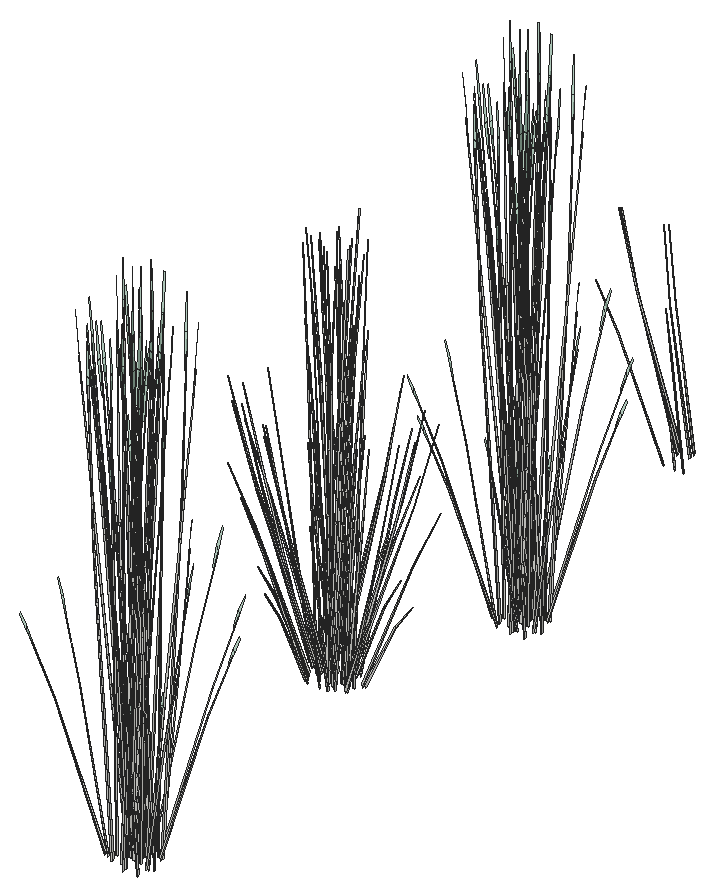
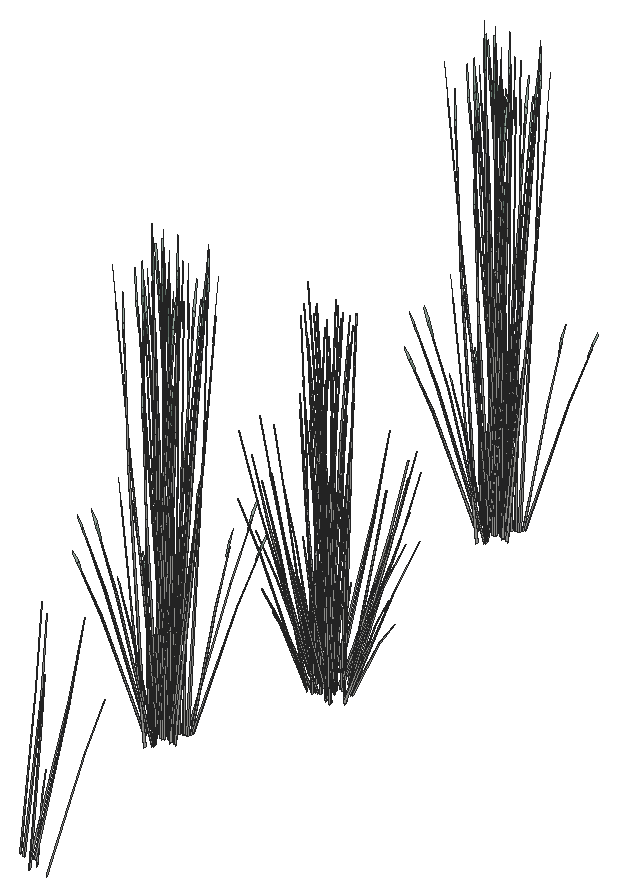
# SketchUp Ruby script. Lengths in inches.
U = 1.inch
M = Sketchup.active_model
def pt(a) = Geom::Point3d.new(a.map { |v| v * U })
def face(e, loops, mat)
  f = e.add_face(loops[0].map { |a| pt(a) })
  loops[1..].each { |l| e.add_face(l.map { |a| pt(a) }).erase! }
  f.material = f.back_material = mat if mat
  f
end
# faces: each face lists its corners as indices into pts; further lists are holes
def faces(e, pts, list, mat = nil) = list.each { |f| face(e, (f[0].is_a?(Array) ? f : [f]).map { |l| l.map { |i| pts[i] } }, mat) }
# xy, xz, yz: faces in a plane at the given z, y or x. An outline is a flat list of corners, or four numbers for a rectangle; further outlines are holes
def ring(l) = l.size == 4 ? [[l[0], l[1]], [l[2], l[1]], [l[2], l[3]], [l[0], l[3]]] : l.each_slice(2).to_a
def flat(e, list, mat, &to3) = list.each { |f| face(e, (f[0].is_a?(Array) ? f : [f]).map { |l| ring(l).map { |u, v| to3.(u, v) } }, mat) }
def xy(e, z, list, mat = nil) = flat(e, list, mat) { |x, y| [x, y, z] }
def xz(e, y, list, mat = nil) = flat(e, list, mat) { |x, z| [x, y, z] }
def yz(e, x, list, mat = nil) = flat(e, list, mat) { |y, z| [x, y, z] }
def lines(e, pts, list) = list.each { |a, b| e.add_line(pt(pts[a]), pt(pts[b])) }
# prism: a flat outline (further loops are holes) pulled along v
def prism(e, loops, v, mat = nil)
  f = face(e, loops, mat); d = Geom::Vector3d.new(v.map { |x| x * U })
  f.pushpull(f.normal.samedirection?(d) ? d.length : -d.length)
end
def box(e, o, s, mat = nil) = prism(e, [[o, [o[0] + s[0], o[1], o[2]], [o[0] + s[0], o[1] + s[1], o[2]], [o[0], o[1] + s[1], o[2]]]], [0, 0, s[2]], mat)
def at(x, y, z, deg = 0) = Geom::Transformation.translation(pt([x, y, z])) * Geom::Transformation.rotation(ORIGIN, Z_AXIS, deg.degrees)
def axes(o, x, y, z) = Geom::Transformation.new([*x, 0, *y, 0, *z, 0, *pt(o).to_a, 1])
def part(name) = M.definitions.add(name)
# library, detail: a bought-in or finely detailed component or shape, given as its bounding box
def library(name, o, s) = part(name).tap { |d| box(d.entities, o, s) }
def detail(e, o, s) = box(e.add_group.entities, o, s)
def put(e, d, t, mat = nil) = e.add_instance(d, t).tap { |i| i.material = mat if mat }
def group(e, t, mat = nil) = e.add_group.tap { |g| g.transformation = t; g.material = mat if mat }.entities
root = M.entities
M.materials.add("LightPink_Translucent").color = [175, 214, 192]
M.materials["LightPink_Translucent"].alpha = 0.75
c1 = part("blade")
p = [[2.15,0.21,22],[0,0.17,0],[0.09,0.45,0],[2.18,0.31,22],[2.29,0.31,22],[0.38,0.45,0],
  [2.48,0.24,33],[2.49,0.24,33],[2.48,0.22,33]]
faces(c1.entities,p,[[0,1,2,3],[4,5,2,3],[6,3,4,7],[8,0,3,6]])
c2 = part("seeds")
p = [[0.3,-0.1,1.38],[-0.01,-0.03,1.59],[-0.01,-0.03,0.03],[0.14,-0.07,-0.07],[0.29,-0.03,3],[0.15,0.01,3.11]]
faces(c2.entities,p,[[0,1,2,3],[1,0,4,5]],"LightPink_Translucent")
c3 = part("blade with seeds")
put(c3.entities,c1,at(0,0,0))
put(c3.entities,c2,axes([2.4,0.25,30.99],[1.5799,-0.05474,1.17369],[-0.12525,1.92788,0.29478],[-0.07173,-0.02425,1.56792]))
c4 = part("blade with seeds\#1")
put(c4.entities,c1,at(0,0,0))
put(root,c3,axes([491.39,414.54,139.33],[-0.44625,-0.29882,0],[0.24886,-0.49993,-0.46963],[0.05668,-0.11386,1.48977]))
put(root,c3,axes([490.75,414,139.53],[0.07025,0.15082,1.30132],[-0.21183,0.37238,-0.27986],[-0.18329,-0.11083,0.55638]))
put(root,c3,axes([494.75,413.78,139.11],[-0.36364,-0.13787,-0.03542],[0.11186,-0.42434,-0.16061],[0.05948,-0.06443,0.52975]))
put(root,c3,axes([495.21,414.42,139.53],[-0.14568,-0.02894,1.30132],[-0.12195,-0.4231,-0.27986],[0.1883,-0.0989,0.55638]))
put(root,c3,axes([493.09,413.55,139.33],[0,-0.59763,0],[0.49772,0,-0.46963],[0.11336,0,1.48977]))
put(root,c3,axes([493.23,414.02,139.29],[-0.37441,-0.44456,0.27988],[0.37047,-0.44483,-0.33208],[0.10632,-0.01552,1.50045]))
put(root,c3,axes([492.3125,416.03,139.41],[0.35844,-0.4667,-0.22925],[0.40249,0.39271,0.50168],[-0.04193,-0.12567,1.53076]))
put(root,c3,axes([491.63,414.8,139.43],[-0.22267,0.44731,0.45182],[-0.39927,-0.26736,0],[0.05071,-0.10188,1.43328]))
put(root,c3,axes([492.44,415.22,139.39],[0.5277,0.12668,-0.2132],[-0.09198,0.60063,0.46656],[0.07287,-0.10495,1.42361]))
put(root,c3,axes([492.32,415.44,139.55],[-0.39744,-0.0922,0.13176],[0.06899,-0.45047,-0.37626],[0.04081,-0.08198,1.15337]))
put(root,c3,axes([493.02,413.92,139.43],[-0.44533,0,0.45182],[0,-0.53472,0],[0.10143,0,1.43328]))
put(root,c3,axes([491.33,416.37,139.17],[0.44781,-0.29509,-0.04679],[0.24886,0.49993,0.46963],[-0.04264,-0.12319,1.48904]))
put(root,c3,axes([491.09,414.1,139.74],[0.07886,0.43418,0.05922],[-0.31771,0.09982,-0.78537],[-0.16083,-0.02753,0.70398]))
put(root,c3,axes([495.22,415.42,139.11],[-0.25548,-0.33028,-0.03542],[0.27981,-0.30262,-0.16061],[0.07928,-0.02131,0.52975]))
put(root,c3,axes([492.7,415.29,139.32],[-0.09383,0.60408,0.41637],[-0.52992,-0.12294,0.16339],[0.05117,-0.08828,1.44559]))
put(root,c3,axes([491.85,414.97,139.42],[0.1182,0.51358,0.16054],[-0.43988,0.12682,0.31929],[0.06409,-0.0458,1.4597]))
put(root,c3,axes([491.78,415.63,139.17],[0.19993,-0.48183,0],[0.41543,0.23189,0],[0,0,1.48063]))
put(root,c3,axes([491.28,416.74,139.33],[-0.44625,0.29882,0],[-0.24886,-0.49993,-0.46963],[-0.05668,-0.11386,1.48977]))
put(root,c3,axes([491.83,416.49,139.42],[0.44258,0.13807,0.16054],[-0.12525,0.50524,0.31929],[-0.00216,-0.08728,1.4597]))
put(root,c3,axes([492.42,416.26,139.55],[-0.26757,0.3531,0.13176],[-0.30187,-0.29453,-0.37626],[-0.04081,-0.08198,1.15337]))
put(root,c3,axes([492.75,416.14,139.26],[0.3833,-0.44456,-0.05579],[0.38354,0.44483,0],[0.01339,-0.01552,1.5977]))
put(root,c3,axes([491.5625,416.38,139.29],[-0.14475,0.59835,0.27988],[-0.51739,-0.14969,-0.33208],[-0.06475,-0.09903,1.50045]))
put(root,c3,axes([491.59,416.64,139.43],[0.22267,0.44731,0.45182],[-0.39927,0.26736,0],[-0.05071,-0.10188,1.43328]))
put(root,c3,axes([493.1875,415.24,139.32],[-0.49797,0.2078,0.41637],[-0.17316,-0.59373,0.16339],[0.0915,0.00726,1.44559]))
put(root,c3,axes([491.96,415.74,139.18],[0.38394,-0.15594,0],[0.13445,0.4453,0],[0,0,1.40478]))
put(root,c3,axes([492.96,417.28,139.42],[0.32439,-0.37551,0.16054],[0.31463,0.37842,0.31929],[-0.06625,-0.04147,1.4597]))
put(root,c3,axes([493.14,415.99,139.18],[0.51528,0,0],[0,0.59763,0],[0,0,1.63305]))
put(root,c3,axes([493.05,415.43,139.38],[-0.21584,0.53851,0.21899],[-0.44849,-0.25917,0.45502],[0.10338,0,1.46094]))
put(root,c3,axes([492.9375,416.29,139.26],[-0.51503,0,-0.0513],[0,-0.59763,0],[-0.01619,0,1.63225]))
put(root,c3,axes([494.13,415.01,139.42],[-0.44258,-0.13807,0.16054],[0.12525,-0.50524,0.31929],[0.00216,0.08728,1.4597]))
put(root,c3,axes([491.94,416,139.25],[-0.51161,0.2078,-0.05471],[-0.17927,-0.59373,0],[-0.01787,0.00726,1.56677]))
put(root,c3,axes([494.68,414.77,139.33],[0.44625,-0.29882,0],[0.24886,0.49993,-0.46963],[0.05668,0.11386,1.48977]))
put(root,c3,axes([492.61,417.72,139.17],[0.00356,-0.59734,-0.04529],[0.49772,0,0.45448],[-0.1133,-0.01877,1.441]))
put(root,c3,axes([494.11,416.54,139.42],[-0.1182,-0.51358,0.16054],[0.43988,-0.12682,0.31929],[-0.06409,0.0458,1.4597]))
put(root,c3,axes([493.47,415.7,139.32],[-0.40415,-0.39628,0.41637],[0.35675,-0.4708,0.16339],[0.04033,0.09554,1.44559]))
put(root,c3,axes([492.83,416.38,139.19],[-0.28765,0.33362,0],[-0.28765,-0.33362,0],[0,0,1.54032]))
put(root,c3,axes([491.77,416.17,139.18],[-0.19993,0.48183,0],[-0.41543,-0.23189,0],[0,0,1.59208]))
put(root,c3,axes([493.26,416.22,139.34],[0.09383,-0.60408,0.44771],[0.52992,0.12294,0.17569],[-0.05117,0.08828,1.5544]))
put(root,c3,axes([493.03,416.39,139.18],[0,0.53472,0],[-0.46104,0,0],[0,0,1.6235]))
put(root,c3,axes([493.08,416.58,139.55],[0.12987,0.4453,0.13176],[-0.37086,0.15594,-0.37626],[-0.08162,0,1.15337]))
put(root,c3,axes([495.04,416.52,139.53],[-0.09014,-0.13585,1.30132],[0.15777,-0.40687,-0.27986],[0.19621,0.07542,0.55638]))
put(root,c3,axes([492.94,417.59,139.43],[0.44533,0,0.45182],[0,0.53472,0],[-0.10143,0,1.43328]))
put(root,c3,axes([493.64,416.07,139.55],[0.39744,0.0922,0.13176],[-0.06899,0.45047,-0.37626],[-0.04081,0.08198,1.15337]))
put(root,c3,axes([494.34,416.71,139.43],[0.22267,-0.44731,0.45182],[0.39927,0.26736,0],[-0.05071,0.10188,1.43328]))
put(root,c3,axes([492.01,416.32,139.16],[0.1511,0.50177,-0.1747],[-0.43526,0.17632,0.00007],[0.0167,0.05539,1.58246]))
put(root,c3,axes([491.74,416.18,139.53],[0.14762,0.00843,1.30132],[0.1649,0.40305,-0.27986],[-0.17669,0.12442,0.55638]))
put(root,c3,axes([492.87,417.96,139.33],[0,0.59763,0],[-0.49772,0,-0.46963],[-0.11336,0,1.48977]))
put(root,c3,axes([494.57,416.97,139.33],[0.44625,0.29882,0],[-0.24886,0.49993,-0.46963],[-0.05668,0.11386,1.48977]))
put(root,c3,axes([493.18,418.71,139.23],[0.28477,-0.29631,-0.05904],[0.26092,0.32453,-0.26768],[0.01837,0.09195,0.88292]))
put(root,c3,axes([493.98,417.83,139.53],[0.01319,-0.17074,1.30132],[0.35385,-0.17492,-0.27986],[0.1001,0.20976,0.55638]))
put(root,c3,axes([492.8,418.14,138.97],[-0.05344,-0.30783,1.28841],[0.4254,-0.049,0.07375],[0.06439,0.2156,0.73315]))
put(root,c3,axes([492.17,418.23,139.53],[0.10953,-0.1151,1.30132],[0.36232,0.14976,-0.27986],[-0.04908,0.23288,0.55638]))
put(root,c4,axes([487.07,449.72,138.84],[-0.14131,0.07713,1.17311],[-0.4232,-0.13499,-0.25229],[0.07845,-0.16789,0.50157]))
put(root,c4,axes([486.43,449.99,140.8],[-0.23727,-0.30983,-0.58282],[0.48842,-0.17267,0.07033],[-0.05548,-0.1497,0.82446]))
put(root,c4,axes([484.89,449.57,138.84],[-0.0301,0.12465,1.17311],[-0.44009,0.10435,-0.25229],[-0.10287,-0.16111,0.50157]))
put(root,c4,axes([487.42,450.29,140.8],[0.01294,-0.35246,-0.58282],[0.54471,0.02367,0.07033],[0.05748,-0.14932,0.82446]))
put(root,c4,axes([486.55,449.1,138.99],[0.06377,0.2222,0.94226],[-0.35378,-0.12306,0.69231],[0.03807,-0.11377,0.20754]))
put(root,c4,axes([486.25,449.92,140.56],[-0.48869,-0.09552,-0.41919],[0.16751,-0.3275,-0.3247],[-0.04481,-0.13186,0.80208]))
put(root,c4,axes([487.31,450.17,140.56],[-0.35588,-0.25603,-0.41919],[0.37594,-0.22422,-0.3247],[0.05415,-0.13008,0.80208]))
put(root,c4,axes([484.73,449.37,138.99],[0.25932,0.13262,0.94226],[-0.37767,0.07972,0.69231],[-0.08081,-0.10192,0.20754]))
put(root,c4,axes([485.36,450.07,140.8],[-0.4239,-0.18418,-0.58282],[0.30126,-0.32274,0.07033],[-0.15358,-0.10997,0.82446]))
put(root,c4,axes([485.16,450.08,140.56],[-0.49056,0.09058,-0.41919],[-0.08581,-0.34303,-0.3247],[-0.13176,-0.0983,0.80208]))
put(root,c4,axes([488.05,450.76,140.56],[-0.12771,-0.34793,-0.41919],[0.48364,-0.06086,-0.3247],[0.1386,-0.09345,0.80208]))
put(root,c4,axes([488.06,450.9,140.8],[0.25968,-0.30066,-0.58282],[0.45504,0.21367,0.07033],[0.15505,-0.10893,0.82446]))
put(root,c4,axes([488.43,450.625,138.84],[-0.1776,-0.01129,1.17311],[-0.18194,-0.30276,-0.25229],[0.21818,-0.08565,0.50157]))
put(root,c4,axes([488.64,450.07,138.99],[-0.16559,0.19397,0.94226],[-0.14233,-0.26061,0.69231],[0.13676,-0.0653,0.20754]))
put(root,c4,axes([484.09,450.625,138.84],[0.09706,0.10609,1.17311],[-0.22366,0.28837,-0.25229],[-0.22965,-0.06892,0.50157]))
put(root,c4,axes([484.5,450.53,140.8],[-0.49695,-0.00917,-0.58282],[0.03338,-0.38634,0.07033],[-0.21053,-0.04077,0.82446]))
put(root,c4,axes([484.33,450.61,140.56],[-0.36098,0.25241,-0.41919],[-0.31614,-0.26664,-0.3247],[-0.18341,-0.0384,0.80208]))
put(root,c4,axes([485.94,451.42,138.71],[0.56014,0.18468,0.19741],[-0.26958,0.38374,0.41019],[0,-0.08846,1.31701]))
put(root,c4,axes([483.52,450.94,138.99],[0.31739,-0.02727,0.94226],[-0.20133,0.24024,0.69231],[-0.15684,-0.03604,0.20754]))
put(root,c4,axes([485.76,451.16,138.95],[-0.53984,0.02352,0.36702],[-0.04882,-0.39046,-0.17663],[0.09664,-0.03957,1.17838]))
put(root,c4,axes([484.37,451.45,138.75],[0,0.38104,0.40731],[-0.5562,0,0],[0,-0.08679,1.29208]))
put(root,c4,axes([485.74,451.31,138.65],[0.21614,0.42608,0.37535],[-0.61757,0.14817,0.14729],[0.00755,-0.07829,1.30318]))
put(root,c4,axes([488.27,451.53,140.56],[0.13468,-0.34661,-0.41919],[0.46175,0.1188,-0.3247],[0.18591,-0.03178,0.80208]))
put(root,c4,axes([487.27,450.32,138.75],[-0.46527,-0.19052,0.40731],[0.2781,-0.34163,0],[0.10597,0.04339,1.29208]))
put(root,c4,axes([485.63,451.64,138.95],[-0.2412,0.34335,0.36702],[-0.50118,-0.16524,-0.17663],[0,-0.07915,1.17838]))
put(root,c4,axes([486.22,451.0625,138.65],[-0.41219,0.3458,0.37535],[-0.4897,-0.30525,0.14729],[0.09937,-0.03451,1.30318]))
put(root,c4,axes([485.51,450.49,138.75],[-0.14361,0.37869,0.14473],[-0.52552,-0.10717,0.28783],[0.09078,-0.00184,1.3159]))
put(root,c4,axes([488.18,451.66,140.8],[0.43684,-0.16829,-0.58282],[0.24345,0.34641,0.07033],[0.21107,-0.03935,0.82446]))
put(root,c4,axes([486.61,450.92,138.86],[0.0959,-0.34006,0.11878],[0.46856,0.05903,-0.33919],[0.08527,0.03492,1.03975]))
put(root,c4,axes([486.41,451,138.95],[-0.29864,-0.31983,0.36702],[0.45236,-0.22522,-0.17663],[0.09664,0.03957,1.17838]))
put(root,c4,axes([485.8,451.72,138.65],[0.62833,0.08028,0.37535],[-0.12787,0.45342,0.14729],[-0.09182,-0.04378,1.30318]))
put(root,c4,axes([487.1,450.52,138.75],[-0.5342,0.10113,0.14473],[-0.13191,-0.37638,0.28783],[0.04764,0.05484,1.3159]))
put(root,c4,axes([485.46,452.45,138.75],[0.5342,-0.10113,0.14473],[0.13191,0.37638,0.28783],[-0.04764,-0.05484,1.3159]))
put(root,c4,axes([486.76,451.24,138.67],[-0.62833,-0.08028,0.4036],[0.12787,-0.45342,0.15838],[0.09182,0.04378,1.40127]))
put(root,c4,axes([485.95,452.05,138.86],[-0.0959,0.34006,0.11878],[-0.46856,-0.05903,-0.33919],[-0.08527,-0.03492,1.03975]))
put(root,c4,axes([487.87,451.5,138.75],[-0.39059,-0.27756,0.14473],[0.39362,-0.26921,0.28783],[-0.04314,0.05668,1.3159]))
put(root,c4,axes([484.96,451.15,139.46],[0.14131,-0.05512,1.45254],[0.04873,0.38487,0.11368],[-0.30608,0.05107,0.51915]))
put(root,c4,axes([489.43,451.76,138.99],[-0.30716,0.06291,0.94226],[0.14458,-0.25998,0.69231],[0.16295,0.01779,0.20754]))
put(root,c4,axes([487.05,452.47,138.75],[0.14361,-0.37869,0.14473],[0.52552,0.10717,0.28783],[-0.09078,0.00184,1.3159]))
put(root,c4,axes([486.92,451.32,138.95],[0.2412,-0.34335,0.36702],[0.50118,0.16524,-0.17663],[0,0.07915,1.17838]))
put(root,c4,axes([485.28,452.64,138.75],[0.46527,0.19052,0.40731],[-0.2781,0.34163,0],[-0.10597,-0.04339,1.29208]))
put(root,c4,axes([483.98,451.36,140.56],[-0.13468,0.34661,-0.41919],[-0.46175,-0.1188,-0.3247],[-0.18591,0.03178,0.80208]))
put(root,c4,axes([488.1875,451.51,138.75],[0,-0.38104,0.40731],[0.5562,0,0],[0,0.08679,1.29208]))
put(root,c4,axes([487.13,451.4,138.86],[0.46318,-0.11112,0.11878],[0.1622,0.31732,-0.33919],[0,0.06984,1.03975]))
put(root,c4,axes([486.8,451.8,138.95],[0.53984,-0.02352,0.36702],[0.04882,0.39046,-0.17663],[-0.09664,0.03957,1.17838]))
put(root,c4,axes([488.85,452.17,138.84],[-0.11973,-0.09372,1.17311],[0.15578,-0.31002,-0.25229],[0.24224,0.042,0.50157]))
put(root,c4,axes([486.8,451.97,138.86],[0.36728,0.22894,0.11878],[-0.30636,0.25829,-0.33919],[-0.08527,0.03492,1.03975]))
put(root,c4,axes([487.76,452.36,140.8],[0.49695,0.00917,-0.58282],[-0.03338,0.38634,0.07033],[0.21053,0.04077,0.82446]))
put(root,c4,axes([487.2,452.67,138.75],[0.46527,-0.19052,0.40731],[0.2781,0.34163,0],[-0.10597,0.04339,1.29208]))
put(root,c4,axes([483.43,452.17,138.84],[0.17277,0.03128,1.17311],[0.11135,0.3195,-0.25229],[-0.23468,0.05981,0.50157]))
put(root,c4,axes([483.07,452.84,138.99],[0.20718,-0.1727,0.94226],[0.08175,0.27339,0.69231],[-0.14972,0.04895,0.20754]))
put(root,c4,axes([487.72,452.66,138.99],[-0.27991,-0.10956,0.94226],[0.36143,-0.11132,0.69231],[0.09749,0.0943,0.20754]))
put(root,c4,axes([484.21,452.13,140.56],[0.12771,0.34793,-0.41919],[-0.48364,0.06086,-0.3247],[-0.1386,0.09345,0.80208]))
put(root,c4,axes([487.04,451.42,139.05],[-0.01358,-0.35877,1.15892],[0.61462,0.093,0.4907],[-0.14537,0.19631,1.09393]))
put(root,c4,axes([487.09,452.81,140.56],[0.49056,-0.09058,-0.41919],[0.08581,0.34303,-0.3247],[0.13176,0.0983,0.80208]))
put(root,c4,axes([487.77,453.16,138.91],[-0.31879,-0.01195,0.86186],[0.21053,-0.25381,0.47585],[0.12594,0.09017,0.67605]))
put(root,c4,axes([486.73,452.54,138.84],[0.00877,-0.12631,1.17311],[0.41923,-0.14109,-0.25229],[0.12942,0.15118,0.50157]))
put(root,c4,axes([484.82,453.59,138.99],[-0.01287,-0.22657,0.94226],[0.32149,0.1616,0.69231],[-0.06323,0.10799,0.20754]))
put(root,c4,axes([486,452.97,140.56],[0.48869,0.09552,-0.41919],[-0.16751,0.3275,-0.3247],[0.04481,0.13186,0.80208]))
put(root,c4,axes([484.56,453.1,139.03],[0.45162,-0.06748,0.05338],[0.10383,0.27185,-0.708],[-0.02863,0.13761,0.63462]))
put(root,c4,axes([484.83,452.6,141.1],[-0.01294,0.35246,-0.64693],[-0.54471,-0.02367,0.07807],[-0.05748,0.14932,0.91515]))
put(root,c4,axes([485.82,452.9,140.8],[0.23727,0.30983,-0.58282],[-0.48842,0.17267,0.07033],[0.05548,0.1497,0.82446]))
put(root,c4,axes([484.45,453.39,138.84],[0.15688,-0.06011,1.17311],[0.38733,0.18125,-0.25229],[-0.11528,0.15683,0.50157]))
put(root,c3,axes([492.18,466.59,139.53],[-0.03656,0.1661,1.30132],[-0.37341,0.10705,-0.27986],[-0.0699,-0.22562,0.55638]))
put(root,c3,axes([493.98,467.23,139.53],[-0.12399,0.09331,1.30132],[-0.33702,-0.21502,-0.27986],[0.08055,-0.22079,0.55638]))
put(root,c3,axes([491.39,468.11,139.33],[-0.44625,-0.29882,0],[0.24886,-0.49993,-0.46963],[0.05668,-0.11386,1.48977]))
put(root,c3,axes([490.75,467.57,139.53],[0.07025,0.15082,1.30132],[-0.21183,0.37238,-0.27986],[-0.18329,-0.11083,0.55638]))
put(root,c3,axes([494.75,467.36,139.11],[-0.36364,-0.13787,-0.03542],[0.11186,-0.42434,-0.16061],[0.05948,-0.06443,0.52975]))
put(root,c3,axes([495.21,467.99,139.53],[-0.14568,-0.02894,1.30132],[-0.12195,-0.4231,-0.27986],[0.1883,-0.0989,0.55638]))
put(root,c3,axes([493.09,467.13,139.33],[0,-0.59763,0],[0.49772,0,-0.46963],[0.11336,0,1.48977]))
put(root,c3,axes([493.23,467.59,139.29],[-0.37441,-0.44456,0.27988],[0.37047,-0.44483,-0.33208],[0.10632,-0.01552,1.50045]))
put(root,c3,axes([492.3125,469.6,139.41],[0.35844,-0.4667,-0.22925],[0.40249,0.39271,0.50168],[-0.04193,-0.12567,1.53076]))
put(root,c3,axes([491.63,468.37,139.43],[-0.22267,0.44731,0.45182],[-0.39927,-0.26736,0],[0.05071,-0.10188,1.43328]))
put(root,c3,axes([492.44,468.79,139.39],[0.5277,0.12668,-0.2132],[-0.09198,0.60063,0.46656],[0.07287,-0.10495,1.42361]))
put(root,c3,axes([492.32,469.01,139.55],[-0.39744,-0.0922,0.13176],[0.06899,-0.45047,-0.37626],[0.04081,-0.08198,1.15337]))
put(root,c3,axes([493.02,467.49,139.43],[-0.44533,0,0.45182],[0,-0.53472,0],[0.10143,0,1.43328]))
put(root,c3,axes([491.33,469.94,139.17],[0.44781,-0.29509,-0.04679],[0.24886,0.49993,0.46963],[-0.04264,-0.12319,1.48904]))
put(root,c3,axes([491.09,467.67,139.74],[0.07886,0.43418,0.05922],[-0.31771,0.09982,-0.78537],[-0.16083,-0.02753,0.70398]))
put(root,c3,axes([495.22,469,139.11],[-0.25548,-0.33028,-0.03542],[0.27981,-0.30262,-0.16061],[0.07928,-0.02131,0.52975]))
put(root,c3,axes([492.7,468.86,139.32],[-0.09383,0.60408,0.41637],[-0.52992,-0.12294,0.16339],[0.05117,-0.08828,1.44559]))
put(root,c3,axes([491.85,468.54,139.42],[0.1182,0.51358,0.16054],[-0.43988,0.12682,0.31929],[0.06409,-0.0458,1.4597]))
put(root,c3,axes([491.78,469.2,139.17],[0.19993,-0.48183,0],[0.41543,0.23189,0],[0,0,1.48063]))
put(root,c3,axes([491.28,470.32,139.33],[-0.44625,0.29882,0],[-0.24886,-0.49993,-0.46963],[-0.05668,-0.11386,1.48977]))
put(root,c3,axes([491.83,470.07,139.42],[0.44258,0.13807,0.16054],[-0.12525,0.50524,0.31929],[-0.00216,-0.08728,1.4597]))
put(root,c3,axes([492.42,469.83,139.55],[-0.26757,0.3531,0.13176],[-0.30187,-0.29453,-0.37626],[-0.04081,-0.08198,1.15337]))
put(root,c3,axes([492.75,469.71,139.26],[0.3833,-0.44456,-0.05579],[0.38354,0.44483,0],[0.01339,-0.01552,1.5977]))
put(root,c3,axes([491.5625,469.95,139.29],[-0.14475,0.59835,0.27988],[-0.51739,-0.14969,-0.33208],[-0.06475,-0.09903,1.50045]))
put(root,c3,axes([491.59,470.21,139.43],[0.22267,0.44731,0.45182],[-0.39927,0.26736,0],[-0.05071,-0.10188,1.43328]))
put(root,c3,axes([493.1875,468.8125,139.32],[-0.49797,0.2078,0.41637],[-0.17316,-0.59373,0.16339],[0.0915,0.00726,1.44559]))
put(root,c3,axes([491.96,469.3125,139.18],[0.38394,-0.15594,0],[0.13445,0.4453,0],[0,0,1.40478]))
put(root,c3,axes([492.96,470.86,139.42],[0.32439,-0.37551,0.16054],[0.31463,0.37842,0.31929],[-0.06625,-0.04147,1.4597]))
put(root,c3,axes([493.14,469.56,139.18],[0.51528,0,0],[0,0.59763,0],[0,0,1.63305]))
put(root,c3,axes([493.05,469,139.38],[-0.21584,0.53851,0.21899],[-0.44849,-0.25917,0.45502],[0.10338,0,1.46094]))
put(root,c3,axes([492.9375,469.86,139.26],[-0.51503,0,-0.0513],[0,-0.59763,0],[-0.01619,0,1.63225]))
put(root,c3,axes([494.13,468.59,139.42],[-0.44258,-0.13807,0.16054],[0.12525,-0.50524,0.31929],[0.00216,0.08728,1.4597]))
put(root,c3,axes([491.94,469.57,139.25],[-0.51161,0.2078,-0.05471],[-0.17927,-0.59373,0],[-0.01787,0.00726,1.56677]))
put(root,c3,axes([494.68,468.34,139.33],[0.44625,-0.29882,0],[0.24886,0.49993,-0.46963],[0.05668,0.11386,1.48977]))
put(root,c3,axes([492.61,471.29,139.17],[0.00356,-0.59734,-0.04529],[0.49772,0,0.45448],[-0.1133,-0.01877,1.441]))
put(root,c3,axes([494.11,470.12,139.42],[-0.1182,-0.51358,0.16054],[0.43988,-0.12682,0.31929],[-0.06409,0.0458,1.4597]))
put(root,c3,axes([493.47,469.28,139.32],[-0.40415,-0.39628,0.41637],[0.35675,-0.4708,0.16339],[0.04033,0.09554,1.44559]))
put(root,c3,axes([492.83,469.95,139.19],[-0.28765,0.33362,0],[-0.28765,-0.33362,0],[0,0,1.54032]))
put(root,c3,axes([491.77,469.75,139.18],[-0.19993,0.48183,0],[-0.41543,-0.23189,0],[0,0,1.59208]))
put(root,c3,axes([493.26,469.79,139.34],[0.09383,-0.60408,0.44771],[0.52992,0.12294,0.17569],[-0.05117,0.08828,1.5544]))
put(root,c3,axes([493.03,469.97,139.18],[0,0.53472,0],[-0.46104,0,0],[0,0,1.6235]))
put(root,c3,axes([493.08,470.15,139.55],[0.12987,0.4453,0.13176],[-0.37086,0.15594,-0.37626],[-0.08162,0,1.15337]))
put(root,c3,axes([495.04,470.09,139.53],[-0.09014,-0.13585,1.30132],[0.15777,-0.40687,-0.27986],[0.19621,0.07542,0.55638]))
put(root,c3,axes([492.94,471.17,139.43],[0.44533,0,0.45182],[0,0.53472,0],[-0.10143,0,1.43328]))
put(root,c3,axes([493.64,469.64,139.55],[0.39744,0.0922,0.13176],[-0.06899,0.45047,-0.37626],[-0.04081,0.08198,1.15337]))
put(root,c3,axes([494.34,470.28,139.43],[0.22267,-0.44731,0.45182],[0.39927,0.26736,0],[-0.05071,0.10188,1.43328]))
put(root,c3,axes([492.01,469.89,139.16],[0.1511,0.50177,-0.1747],[-0.43526,0.17632,0.00007],[0.0167,0.05539,1.58246]))
put(root,c3,axes([491.74,469.76,139.53],[0.14762,0.00843,1.30132],[0.1649,0.40305,-0.27986],[-0.17669,0.12442,0.55638]))
put(root,c3,axes([492.87,471.53,139.33],[0,0.59763,0],[-0.49772,0,-0.46963],[-0.11336,0,1.48977]))
put(root,c3,axes([494.57,470.54,139.33],[0.44625,0.29882,0],[-0.24886,0.49993,-0.46963],[-0.05668,0.11386,1.48977]))
put(root,c3,axes([493.18,472.28,139.23],[0.28477,-0.29631,-0.05904],[0.26092,0.32453,-0.26768],[0.01837,0.09195,0.88292]))
put(root,c3,axes([493.98,471.4,139.53],[0.01319,-0.17074,1.30132],[0.35385,-0.17492,-0.27986],[0.1001,0.20976,0.55638]))
put(root,c3,axes([492.8,471.72,138.97],[-0.05344,-0.30783,1.28841],[0.4254,-0.049,0.07375],[0.06439,0.2156,0.73315]))
put(root,c3,axes([492.17,471.8,139.53],[0.10953,-0.1151,1.30132],[0.36232,0.14976,-0.27986],[-0.04908,0.23288,0.55638]))
put(root,c4,axes([487.07,498.93,138.84],[-0.14131,0.07713,1.17311],[-0.4232,-0.13499,-0.25229],[0.07845,-0.16789,0.50157]))
put(root,c4,axes([486.43,499.2,140.8],[-0.23727,-0.30983,-0.58282],[0.48842,-0.17267,0.07033],[-0.05548,-0.1497,0.82446]))
put(root,c4,axes([484.89,498.78,138.84],[-0.0301,0.12465,1.17311],[-0.44009,0.10435,-0.25229],[-0.10287,-0.16111,0.50157]))
put(root,c4,axes([487.42,499.5,140.8],[0.01294,-0.35246,-0.58282],[0.54471,0.02367,0.07033],[0.05748,-0.14932,0.82446]))
put(root,c4,axes([486.55,498.3125,138.99],[0.06377,0.2222,0.94226],[-0.35378,-0.12306,0.69231],[0.03807,-0.11377,0.20754]))
put(root,c4,axes([486.25,499.13,140.56],[-0.48869,-0.09552,-0.41919],[0.16751,-0.3275,-0.3247],[-0.04481,-0.13186,0.80208]))
put(root,c4,axes([487.31,499.38,140.56],[-0.35588,-0.25603,-0.41919],[0.37594,-0.22422,-0.3247],[0.05415,-0.13008,0.80208]))
